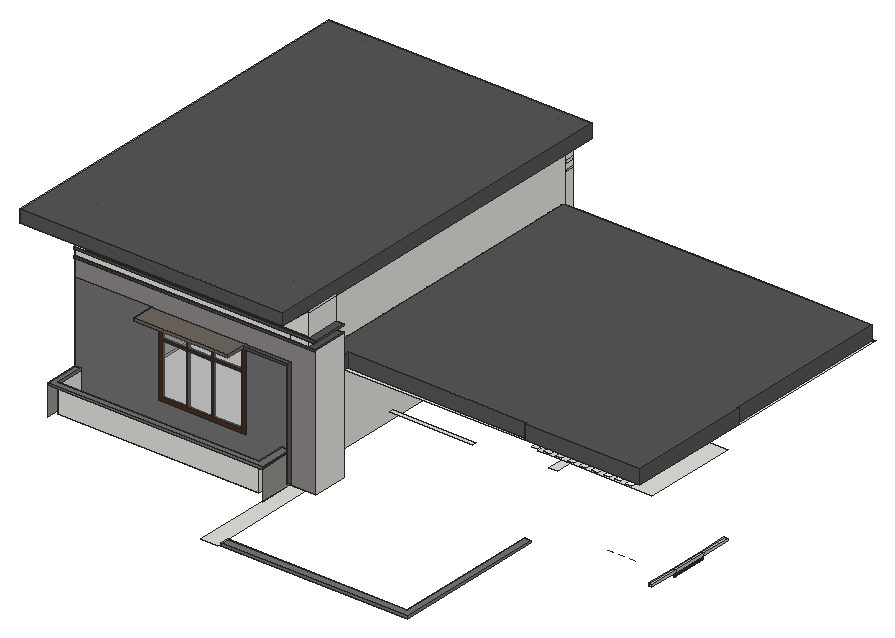
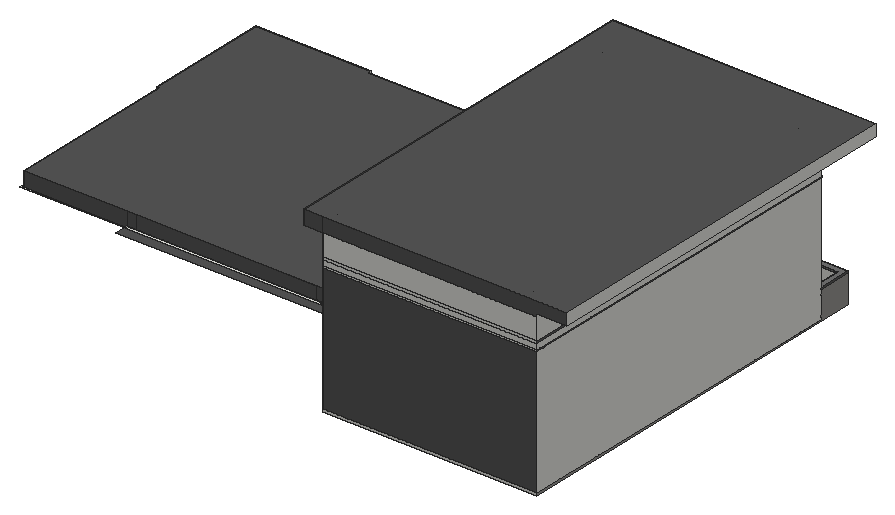
# SketchUp Ruby script. Lengths in inches.
U = 1.inch
M = Sketchup.active_model
def pt(a) = Geom::Point3d.new(a.map { |v| v * U })
def face(e, loops, mat)
  f = e.add_face(loops[0].map { |a| pt(a) })
  loops[1..].each { |l| e.add_face(l.map { |a| pt(a) }).erase! }
  f.material = f.back_material = mat if mat
  f
end
# faces: each face lists its corners as indices into pts; further lists are holes
def faces(e, pts, list, mat = nil) = list.each { |f| face(e, (f[0].is_a?(Array) ? f : [f]).map { |l| l.map { |i| pts[i] } }, mat) }
# xy, xz, yz: faces in a plane at the given z, y or x. An outline is a flat list of corners, or four numbers for a rectangle; further outlines are holes
def ring(l) = l.size == 4 ? [[l[0], l[1]], [l[2], l[1]], [l[2], l[3]], [l[0], l[3]]] : l.each_slice(2).to_a
def flat(e, list, mat, &to3) = list.each { |f| face(e, (f[0].is_a?(Array) ? f : [f]).map { |l| ring(l).map { |u, v| to3.(u, v) } }, mat) }
def xy(e, z, list, mat = nil) = flat(e, list, mat) { |x, y| [x, y, z] }
def xz(e, y, list, mat = nil) = flat(e, list, mat) { |x, z| [x, y, z] }
def yz(e, x, list, mat = nil) = flat(e, list, mat) { |y, z| [x, y, z] }
def lines(e, pts, list) = list.each { |a, b| e.add_line(pt(pts[a]), pt(pts[b])) }
# prism: a flat outline (further loops are holes) pulled along v
def prism(e, loops, v, mat = nil)
  f = face(e, loops, mat); d = Geom::Vector3d.new(v.map { |x| x * U })
  f.pushpull(f.normal.samedirection?(d) ? d.length : -d.length)
end
def box(e, o, s, mat = nil) = prism(e, [[o, [o[0] + s[0], o[1], o[2]], [o[0] + s[0], o[1] + s[1], o[2]], [o[0], o[1] + s[1], o[2]]]], [0, 0, s[2]], mat)
def at(x, y, z, deg = 0) = Geom::Transformation.translation(pt([x, y, z])) * Geom::Transformation.rotation(ORIGIN, Z_AXIS, deg.degrees)
def axes(o, x, y, z) = Geom::Transformation.new([*x, 0, *y, 0, *z, 0, *pt(o).to_a, 1])
def part(name) = M.definitions.add(name)
# library, detail: a bought-in or finely detailed component or shape, given as its bounding box
def library(name, o, s) = part(name).tap { |d| box(d.entities, o, s) }
def detail(e, o, s) = box(e.add_group.entities, o, s)
def put(e, d, t, mat = nil) = e.add_instance(d, t).tap { |i| i.material = mat if mat }
def group(e, t, mat = nil) = e.add_group.tap { |g| g.transformation = t; g.material = mat if mat }.entities
root = M.entities
M.materials.add("[Color C08]").color = [86, 44, 0]
M.materials.add("[Color C08]1").color = [78, 44, 34]
M.materials.add("[Color M00]").color = [255, 255, 255]
M.materials.add("[Color M05]").color = [114, 114, 114]
M.materials.add("[Color M06]").color = [86, 86, 86]
M.materials.add("[Color M07]").color = [58, 58, 58]
M.materials.add("[Granite Light Gray]").color = [149, 148, 144]
M.materials.add("[Metal Corrugated Shiny]").color = [193, 193, 193]
M.materials.add("[Metal Seamed]").color = [118, 119, 115]
M.materials.add("[Roofing Shingles Asphalt]").color = [111, 104, 97]
M.materials.add("[Stone Marble]").color = [143, 138, 136]
M.materials.add("[Translucent Glass Gray]").color = [128, 128, 128]
M.materials["[Translucent Glass Gray]"].alpha = 0.5
c1 = part("Group\#8")
xy(c1.entities,0,[[0,0,93.8125,6]])
xy(c1.entities,4.34,[[4.34,0,30.21,6],[31.52,0,57.71,6],[59.02,0,89.48,6]],"[Color C08]1")
xy(c1.entities,64.91,[[4.34,0,30.21,6],[31.52,0,57.71,6],[59.02,0,89.48,6]],"[Color C08]1")
xy(c1.entities,67.24,[[4.34,0,30.21,6],[31.52,0,57.71,6],[59.02,0,89.48,6]],"[Color C08]1")
xy(c1.entities,89.48,[[4.34,0,30.21,6],[31.52,0,57.71,6],[59.02,0,89.48,6]],"[Color C08]1")
xy(c1.entities,93.8125,[[0,0,93.8125,6]],"[Color C08]1")
xz(c1.entities,0,[[[0,0,93.8125,93.8125],[59.02,4.34,89.48,64.91],[31.52,4.34,57.71,64.91],[4.34,4.34,30.21,64.91],[59.02,67.24,89.48,89.48],[31.52,67.24,57.71,89.48],[4.34,67.24,30.21,89.48]]],"[Color C08]1")
xz(c1.entities,0,[[4.34,4.34,30.21,64.91],[31.52,4.34,57.71,64.91],[59.02,4.34,89.48,64.91],[4.34,67.24,30.21,89.48],[31.52,67.24,57.71,89.48],
  [59.02,67.24,89.48,89.48]],"[Translucent Glass Gray]")
xz(c1.entities,6,[[[0,0,93.8125,93.8125],[59.02,4.34,89.48,64.91],[31.52,4.34,57.71,64.91],[4.34,4.34,30.21,64.91],[59.02,67.24,89.48,89.48],[31.52,67.24,57.71,89.48],[4.34,67.24,30.21,89.48]]],"[Color C08]1")
yz(c1.entities,0,[[0,0,6,93.8125]],"[Color C08]1")
yz(c1.entities,4.34,[[0,4.34,6,64.91],[0,67.24,6,89.48]],"[Color C08]1")
yz(c1.entities,30.21,[[0,4.34,6,64.91],[0,67.24,6,89.48]],"[Color C08]1")
yz(c1.entities,31.52,[[0,4.34,6,64.91],[0,67.24,6,89.48]],"[Color C08]1")
yz(c1.entities,57.71,[[0,4.34,6,64.91],[0,67.24,6,89.48]],"[Color C08]1")
yz(c1.entities,59.02,[[0,4.34,6,64.91],[0,67.24,6,89.48]],"[Color C08]1")
yz(c1.entities,89.48,[[0,4.34,6,64.91],[0,67.24,6,89.48]],"[Color C08]1")
yz(c1.entities,93.8125,[[0,0,6,93.8125]],"[Color C08]1")
xy(root,268.48,[[503.61,435.35,506.53,462.36],[503.61,462.36,506.53,494.13],[503.61,494.13,506.53,521]])
xy(root,270.48,[[503.61,435.35,506.53,435.41]])
xy(root,270.48,[[503.61,435.41,506.53,462.36],[503.61,462.36,506.53,494.13],[503.61,494.13,506.53,521]],"[Metal Corrugated Shiny]")
xy(root,276.0625,[[238,280.08,238,287.59,401.36,287.59,401.36,421.2,405.5625,421.2,405.5625,280.08],[405.5625,280.08,407.6875,421.2]])
xy(root,278.0625,[[223,275.76,238,376.79],[223,376.79,238,408.45],[238,376.79,246.5625,408.45]])
xy(root,278.0625,[[238,280.08,407.6875,280.08,407.6875,421.2,401.36,421.2,401.36,287.59,238,287.59]],"[Metal Seamed]")
xy(root,280.375,[[32.29,351.11,215.78,376.79],[223,373.6,224.1875,376.79],[[27.5625,376.79,223,699.87],[38.1875,380.8125,217,690.87]]])
xy(root,305.13,[[103.53,376.79,183.1,380.8125]])
xy(root,306.375,[[27.5625,345.62,223,345.62,223,376.79,215.78,376.79,215.78,351.11,32.29,351.11,32.29,376.79,27.5625,376.79]],"[Color M05]")
xy(root,323.85,[[402.3125,448.18,410.3125,499.8]])
xy(root,337.83,[[279.03,421.2,354.66,424.01]])
xy(root,343.15,[[402.3125,435.41,410.3125,521],[410.3125,435.41,506.53,521]])
xy(root,357.8125,[[223,408.45,223,688.37,504.53,688.37,504.53,534.31,506.53,534.31,506.53,421.2,401.5625,421.2,401.5625,424.01,238,424.01,238,408.45],[411.38,417.2,416.8,421.2],[422.38,417.2,427.8,421.2],[433.38,417.2,438.8,421.2],[444.38,417.2,449.8,421.2],
  [455.38,417.2,460.8,421.2],[466.38,417.2,471.8,421.2],[238,421.2,401.5625,424.01],[504.53,534.31,506.53,688.37],[410.3125,688.37,506.53,690.12]])
xy(root,357.8125,[[477,417.2,482.43,421.2],[487,417.2,492.43,421.2],[497.19,417.2,502.61,421.2]],"[Color M00]")
xy(root,358.9375,[[238,688.37,238,690.87,223,690.87],[238,688.37,410.3125,690.87]])
xy(root,358.9375,[[223,690.87,410.3125,700.56]],"[Color M06]")
xy(root,359,[[223,688.37,238,688.37,223,690.87]])
xy(root,371,[[223,408.45,238,408.45,238,424.01,401.5625,424.01,401.5625,421.2,506.53,421.2,506.53,534.31,504.53,534.31,504.53,688.37,223,688.37]],"[Color M06]")
xy(root,376.51,[[183.1,373.6,223,376.79]],"[Color M06]")
xy(root,376.51,[[96.97,356.72,96.97,376.79,103.53,376.79,103.53,380.8125,183.1,380.8125,183.1,356.72]],"[Roofing Shingles Asphalt]")
xy(root,379.01,[[183.1,373.6,224.1875,376.79]],"[Color M06]")
xy(root,379.01,[[96.97,356.72,183.1,376.79]],"[Roofing Shingles Asphalt]")
xy(root,389.4375,[[38.1875,380.8125,217,690.87]])
xy(root,395.4375,[[38.1875,380.8125,217,690.87]])
xy(root,395.4375,[[27.5625,375.66,246.5625,376.79]],"[Color M06]")
xy(root,396.9375,[[27.5625,375.66,223,376.79],[223,375.66,246.5625,376.79],[240,376.79,246.5625,408.45]],"[Color M06]")
xy(root,402.3125,[[27.5625,375.66,246.5625,376.79],[240,376.79,246.5625,408.45]],"[Color M06]")
xy(root,404.125,[[27.5625,375.66,246.5625,376.79],[240,376.79,246.5625,408.45]],"[Color M06]")
xy(root,424.4375,[[223,376.79,240,408.45],[223,408.45,240,699.87]])
xy(root,426.4375,[[0,348.1,0,699.87,27.5625,699.87,27.5625,376.79,240,376.79,240,348.1],[38.1875,376.79,39.5625,380.8125],[38.1875,380.8125,217,388.69],[38.1875,388.69,217,690.87]])
xy(root,426.4375,[[39.5625,376.79,217,380.8125]],"[Color C08]1")
xy(root,437.4375,[[0,348.1,240,699.87]],"[Color M06]")
xz(root,280.08,[[238,276.0625,407.6875,278.0625]],"[Metal Seamed]")
xz(root,287.59,[[238,276.0625,401.36,278.0625]],"[Metal Seamed]")
xz(root,345.62,[[27.5625,304.375,223,306.375]],"[Color M05]")
xz(root,348.1,[[0,426.4375,240,437.4375]],"[Color M06]")
xz(root,351.11,[[32.29,280.375,215.78,304.375]])
xz(root,351.11,[[32.29,304.375,215.78,306.375]],"[Color M05]")
xz(root,356.72,[[96.97,376.51,183.1,379.01]],"[Roofing Shingles Asphalt]")
xz(root,373.6,[[223,280.375,224.1875,280.375,224.1875,379.01,183.1,379.01,183.1,376.51,223,376.51]],"[Color M06]")
xz(root,375.66,[[27.5625,395.4375,246.5625,396.9375],[27.5625,402.3125,246.5625,404.125]],"[Color M06]")
xz(root,376.79,[[223,278.0625,224.1875,280.375],[27.5625,280.375,32.29,304.375],[215.78,280.375,223,304.375],[223,280.375,224.1875,304.375],[27.5625,304.375,32.29,306.375],
  [215.78,304.375,223,306.375],[223,304.375,224.1875,376.51],[27.5625,396.9375,223,402.3125],[223,396.9375,240,402.3125],[223,402.3125,246.5625,404.125],
  [27.5625,404.125,38.1875,424.4375],[218.09,405,240,424.4375],[218.09,424.4375,240,426.4375]])
xz(root,376.79,[[[38.1875,404.125,217.85,404.125,218.09,405,203.87,405,203.87,424.4375,217,424.4375,217,426.4375,38.1875,426.4375],[167.43,405,185.75,424.4375],[148.74,405,166.3125,424.4375],[130.05,405,147.625,424.4375],[111.37,405,128.9375,424.4375],[92.68,405,110.25,424.4375],[73.99,405,91.5625,424.4375],[55.3,405,72.875,424.4375],[186.87,405,202.75,424.4375],[39.3,405,54.1875,424.4375]],[217,405,218.09,424.4375],[217,424.4375,218.09,426.4375]],"[Color C08]")
xz(root,376.79,[[217.85,404.125,223,404.125,223,405,218.09,405],[223,404.125,240,405],[27.5625,424.4375,38.1875,426.4375]],"[Color M00]")
xz(root,376.79,[[32.29,280.375,215.78,280.375,215.78,306.375,223,306.375,223,376.51,183.1,376.51,183.1,305.13,103.53,305.13,103.53,376.51,96.97,376.51,96.97,379.01,27.5625,379.01,27.5625,306.375,32.29,306.375]],"[Color M05]")
xz(root,376.79,[[224.1875,278.0625,246.5625,278.0625,246.5625,395.4375,27.5625,395.4375,27.5625,379.01,224.1875,379.01]],"[Stone Marble]")
xz(root,376.79,[[39.3,405,54.1875,424.4375],[55.3,405,72.875,424.4375],[73.99,405,91.5625,424.4375],[92.68,405,110.25,424.4375],[111.37,405,128.9375,424.4375],
  [130.05,405,147.625,424.4375],[148.74,405,166.3125,424.4375],[167.43,405,185.75,424.4375],[186.87,405,202.75,424.4375],[203.87,405,217,424.4375]],"[Translucent Glass Gray]")
xz(root,380.8125,[[38.1875,278.375,39.5625,280.375],[39.5625,278.375,217,280.375],[38.1875,280.375,39.5625,389.4375],[[39.5625,280.375,217,389.4375],[103.53,305.13,183.1,376.51]],[38.1875,389.4375,39.5625,395.4375],
  [39.5625,389.4375,217,395.4375],[38.1875,395.4375,39.5625,396.9375],[39.5625,395.4375,217,396.9375],[38.1875,396.9375,39.5625,402.3125],[39.5625,396.9375,217,402.3125],
  [38.1875,402.3125,39.5625,405],[39.5625,402.3125,217,405],[38.1875,405,39.5625,424.4375],[39.5625,405,217,424.4375],[38.1875,424.4375,39.5625,426.4375],
  [39.5625,424.4375,217,426.4375]])
xz(root,408.45,[[223,278.0625,238,357.8125],[238,278.0625,238,371,223,371,223,395.4375,246.5625,395.4375,246.5625,278.0625],[223,357.8125,238,371],[223,405,240,424.4375]])
xz(root,408.45,[[223,395.4375,223,402.3125,240,402.3125,240,396.9375,246.5625,396.9375,246.5625,395.4375],[223,402.3125,223,405,240,405,240,404.125,246.5625,404.125,246.5625,402.3125]],"[Color M06]")
xz(root,421.2,[[401.36,276.0625,401.5625,278.0625],[401.5625,276.0625,407.6875,278.0625]])
xz(root,421.2,[[401.5625,357.8125,506.53,371]],"[Color M06]")
xz(root,424.01,[[238,357.8125,401.5625,371]],"[Color M06]")
xz(root,435.35,[[503.61,268.48,506.53,270.48]])
xz(root,462.36,[[503.61,268.48,506.53,270.48]])
xz(root,521,[[503.61,268.48,506.53,270.48]])
xz(root,534.31,[[504.53,357.8125,506.53,371]])
xz(root,688.37,[[223,357.8125,238,359],[238,357.8125,401.5625,358.9375],[401.5625,357.8125,410.3125,358.9375]])
xz(root,688.37,[[410.3125,357.8125,504.53,371],[238,358.9375,401.5625,371],[401.5625,358.9375,410.3125,371],[223,359,238,371]],"[Color M06]")
xz(root,690.87,[[38.1875,278.375,217,280.375],[38.1875,280.375,217,389.4375],[38.1875,389.4375,217,395.4375],[38.1875,395.4375,217,396.9375],[38.1875,396.9375,217,402.3125],
  [38.1875,402.3125,217,405],[38.1875,405,217,424.4375],[38.1875,424.4375,217,426.4375]])
xz(root,699.87,[[27.5625,278.375,223,280.375],[27.5625,395.4375,223,396.9375],[27.5625,396.9375,223,402.3125],[27.5625,402.3125,223,405],[27.5625,405,223,424.4375]])
xz(root,699.87,[[27.5625,280.375,223,395.4375],[27.5625,424.4375,27.5625,426.4375,0,426.4375,0,437.4375,223,437.4375,223,424.4375],[223,424.4375,240,437.4375]],"[Color M06]")
yz(root,0,[[348.1,426.4375,699.87,437.4375]])
yz(root,27.5625,[[376.79,280.375,699.87,395.4375],[376.79,396.9375,699.87,402.3125],[376.79,405,699.87,426.4375]])
yz(root,27.5625,[[345.62,304.375,376.79,306.375],[375.66,395.4375,699.87,396.9375],[375.66,402.3125,375.66,404.125,376.79,404.125,376.79,405,699.87,405,699.87,402.3125]],"[Color M06]")
yz(root,27.5625,[[345.62,278.375,345.62,304.375,376.79,304.375,376.79,280.375,699.87,280.375,699.87,278.375]],"[Granite Light Gray]")
yz(root,32.29,[[351.11,280.375,376.79,304.375]])
yz(root,32.29,[[351.11,304.375,376.79,306.375]],"[Color M05]")
yz(root,38.1875,[[380.8125,278.375,690.87,280.375],[380.8125,280.375,690.87,389.4375],[380.8125,389.4375,397.5,395.4375],[397.5,389.4375,403.63,395.4375],[403.63,389.4375,690.87,395.4375],
  [380.8125,395.4375,690.87,396.9375],[380.8125,396.9375,690.87,402.3125],[380.8125,402.3125,690.87,405],[380.8125,405,690.87,424.4375],[380.8125,424.4375,690.87,426.4375]])
yz(root,96.97,[[356.72,376.51,376.79,379.01]],"[Roofing Shingles Asphalt]")
yz(root,103.53,[[376.79,305.13,380.8125,376.51]])
yz(root,183.1,[[376.79,305.13,380.8125,376.51]])
yz(root,183.1,[[356.72,376.51,373.6,379.01]],"[Roofing Shingles Asphalt]")
yz(root,215.78,[[351.11,280.375,376.79,304.375]])
yz(root,215.78,[[351.11,304.375,376.79,306.375]],"[Color M05]")
yz(root,217,[[380.8125,278.375,690.87,280.375],[380.8125,280.375,690.87,389.4375],[380.8125,389.4375,690.87,395.4375],[380.8125,395.4375,690.87,396.9375],[380.8125,396.9375,690.87,402.3125],
  [380.8125,402.3125,690.87,405],[380.8125,405,690.87,424.4375],[380.8125,424.4375,690.87,426.4375]])
yz(root,223,[[345.62,278.0625,364.3125,278.375],[364.3125,278.0625,376.79,278.375],[376.79,278.0625,408.45,278.375],[376.79,278.375,408.45,280.375],[373.6,280.375,376.79,306.375],
  [408.45,280.375,688.37,357.8125],[688.37,280.375,690.87,359],[690.87,280.375,699.87,358.9375],[408.45,357.8125,688.37,371],[690.87,358.9375,699.87,395.4375],
  [688.37,359,690.87,359,690.87,424.4375,408.45,424.4375,408.45,371,688.37,371],[690.87,395.4375,699.87,396.9375],[690.87,396.9375,699.87,402.3125],[690.87,402.3125,699.87,405],[690.87,405,699.87,424.4375]])
yz(root,223,[[373.6,306.375,376.79,376.51]],"[Color M06]")
yz(root,223,[[345.62,304.375,373.6,306.375]],"[Color M07]")
yz(root,223,[[345.62,278.375,376.79,278.375,376.79,280.375,373.6,280.375,373.6,304.375,345.62,304.375]],"[Granite Light Gray]")
yz(root,224.1875,[[373.6,280.375,376.79,379.01]],"[Color M06]")
yz(root,238,[[280.08,276.0625,287.59,278.0625]])
yz(root,238,[[408.45,357.8125,421.2,371],[421.2,357.8125,424.01,371]],"[Color M06]")
yz(root,240,[[376.79,396.9375,408.45,402.3125],[376.79,404.125,408.45,424.4375],[376.79,424.4375,408.45,426.4375]])
yz(root,240,[[408.45,424.4375,699.87,424.4375,699.87,437.4375,348.1,437.4375,348.1,426.4375,408.45,426.4375]],"[Color M06]")
yz(root,246.5625,[[376.79,278.0625,408.45,395.4375]])
yz(root,246.5625,[[375.66,395.4375,408.45,396.9375],[375.66,402.3125,376.79,404.125],[376.79,402.3125,408.45,404.125]],"[Color M06]")
yz(root,401.36,[[287.59,276.0625,421.2,278.0625]],"[Metal Seamed]")
yz(root,401.5625,[[421.2,357.8125,424.01,371]])
yz(root,407.6875,[[280.08,276.0625,421.2,278.0625]],"[Metal Seamed]")
yz(root,410.3125,[[688.37,357.8125,690.12,358.9375]])
yz(root,503.61,[[435.35,268.48,435.41,270.48]])
yz(root,503.61,[[435.41,268.48,462.36,270.48],[462.36,268.48,494.13,270.48],[494.13,268.48,521,270.48]],"[Metal Corrugated Shiny]")
yz(root,504.53,[[534.31,357.8125,688.37,371]],"[Color M06]")
yz(root,506.53,[[421.2,357.8125,534.31,371]],"[Color M06]")
yz(root,506.53,[[435.35,268.48,462.36,270.48],[462.36,268.48,494.13,270.48],[494.13,268.48,521,270.48]],"[Metal Corrugated Shiny]")
p = [[505.01,462.36,264.38],[504.84,462.36,264.45],[504.84,494.13,264.45],[505.01,494.13,264.38],[505.18,462.36,264.36],[505.18,494.13,264.36],
  [505.36,462.36,264.38],[505.36,494.13,264.38],[505.53,462.36,264.45],[505.53,494.13,264.45],[504.7,462.36,264.56],[504.7,494.13,264.56],
  [505.67,462.36,264.56],[505.67,494.13,264.56],[504.59,462.36,264.7],[504.59,494.13,264.7],[505.78,462.36,264.7],[505.78,494.13,264.7],
  [504.52,462.36,264.87],[504.52,494.13,264.87],[505.85,462.36,264.87],[505.85,494.13,264.87],[504.5,462.36,265.05],[504.5,494.13,265.05],
  [505.87,462.36,265.05],[505.87,494.13,265.05],[504.52,462.36,265.22],[504.52,494.13,265.22],[505.85,462.36,265.22],[505.85,494.13,265.22],
  [504.59,462.36,265.39],[504.59,494.13,265.39],[505.78,462.36,265.39],[505.78,494.13,265.39],[504.7,462.36,265.53],[504.7,494.13,265.53],
  [505.67,462.36,265.53],[505.67,494.13,265.53],[504.84,462.36,265.64],[504.84,494.13,265.64],[505.53,462.36,265.64],[505.53,494.13,265.64],
  [505.01,462.36,265.71],[505.01,494.13,265.71],[505.36,462.36,265.71],[505.36,494.13,265.71],[505.18,462.36,265.73],[505.18,494.13,265.73],
  [238,688.37,359],[238,688.37,358.9375],[223,690.87,358.9375],[223,690.87,359],[223,376.79,396.9375],[223,408.45,396.9375],
  [492.43,421.2,294.6],[487,421.2,294.6],[502.61,421.2,294.6],[497.19,421.2,294.6],[482.43,421.2,294.6],[477,421.2,294.6],
  [38.1875,690.87,426.4375],[38.1875,690.87,437.4375],[217,690.87,426.4375],[217,690.87,437.4375],[38.1875,388.69,437.4375],[38.1875,388.69,426.4375],
  [217,388.69,437.4375],[217,388.69,426.4375]]
faces(root,p,[[0,1,2,3],[4,0,3,5],[6,4,5,7],[8,6,7,9],[1,10,11,2],[12,8,9,13],[10,14,15,11],[16,12,13,17],
  [14,18,19,15],[20,16,17,21],[18,22,23,19],[24,20,21,25],[22,26,27,23],[28,24,25,29],[26,30,31,27],[32,28,29,33],
  [30,34,35,31],[36,32,33,37],[34,38,39,35],[40,36,37,41],[38,42,43,39],[44,40,41,45],[42,46,47,43],[46,44,45,47]],"[Color M07]")
faces(root,p,[[48,49,50,51]])
lines(root,p,[[52,53],[54,55],[56,57],[58,59],[60,61],[62,63],[64,65],[66,67]])
put(root,c1,axes([103.53,376.79,305.13],[0.8481,0,0],[0,0.28,0],[0,0,0.76384]))
